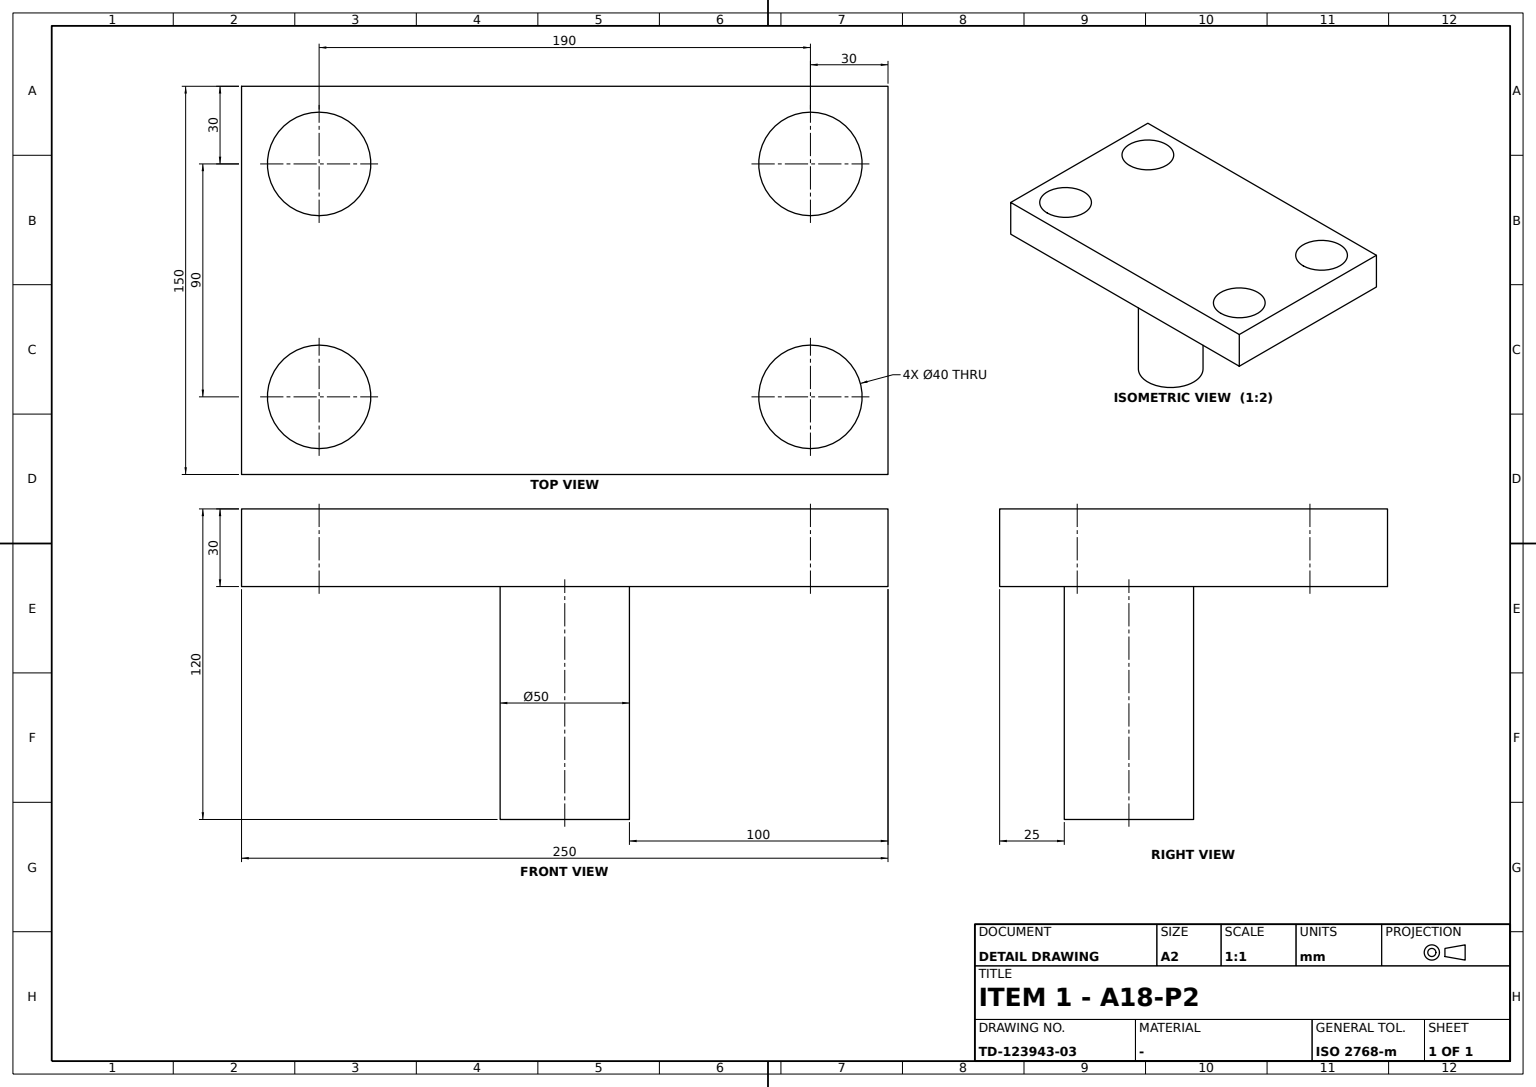
ISO-10303-21;
HEADER;
FILE_DESCRIPTION((''),'2;1');
FILE_NAME('','',(''),(''),'','','');
FILE_SCHEMA(('AUTOMOTIVE_DESIGN'));
ENDSEC;
DATA;
#1=APPLICATION_CONTEXT('');
#2=PRODUCT_CONTEXT('',#1,'mechanical');
#3=PRODUCT('','','',(#2));
#4=PRODUCT_DEFINITION_FORMATION('','',#3);
#5=PRODUCT_DEFINITION_CONTEXT('',#1,'design');
#6=PRODUCT_DEFINITION('','',#4,#5);
#7=PRODUCT_DEFINITION_SHAPE('','',#6);
#8=(LENGTH_UNIT()NAMED_UNIT(*)SI_UNIT(.MILLI.,.METRE.));
#9=(NAMED_UNIT(*)PLANE_ANGLE_UNIT()SI_UNIT($,.RADIAN.));
#10=(NAMED_UNIT(*)SI_UNIT($,.STERADIAN.)SOLID_ANGLE_UNIT());
#11=UNCERTAINTY_MEASURE_WITH_UNIT(LENGTH_MEASURE(0.005),#8,'distance_accuracy_value','');
#12=(GEOMETRIC_REPRESENTATION_CONTEXT(3)GLOBAL_UNCERTAINTY_ASSIGNED_CONTEXT((#11))GLOBAL_UNIT_ASSIGNED_CONTEXT((#8,#9,#10))REPRESENTATION_CONTEXT('',''));
#13=CARTESIAN_POINT('',(65.,95.,-15.));
#14=VERTEX_POINT('',#13);
#15=CARTESIAN_POINT('',(45.,95.,-15.));
#16=DIRECTION('',(0.,0.,1.));
#17=DIRECTION('',(1.,0.,0.));
#18=AXIS2_PLACEMENT_3D('',#15,#16,#17);
#19=CIRCLE('',#18,20.);
#20=EDGE_CURVE('',#14,#14,#19,.F.);
#21=ORIENTED_EDGE('',*,*,#20,.T.);
#22=EDGE_LOOP('',(#21));
#23=FACE_BOUND('',#22,.T.);
#24=CARTESIAN_POINT('',(65.,95.,15.));
#25=VERTEX_POINT('',#24);
#26=CARTESIAN_POINT('',(45.,95.,15.));
#27=AXIS2_PLACEMENT_3D('',#26,#16,#17);
#28=CIRCLE('',#27,20.);
#29=EDGE_CURVE('',#25,#25,#28,.T.);
#30=ORIENTED_EDGE('',*,*,#29,.T.);
#31=EDGE_LOOP('',(#30));
#32=FACE_BOUND('',#31,.T.);
#33=CARTESIAN_POINT('',(45.,95.,14.9));
#34=DIRECTION('',(0.,0.,-1.));
#35=AXIS2_PLACEMENT_3D('',#33,#34,#17);
#36=CYLINDRICAL_SURFACE('',#35,20.);
#37=ADVANCED_FACE('',(#23,#32),#36,.F.);
#38=CARTESIAN_POINT('',(-25.,-95.,15.));
#39=VERTEX_POINT('',#38);
#40=CARTESIAN_POINT('',(-45.,-95.,15.));
#41=AXIS2_PLACEMENT_3D('',#40,#16,#17);
#42=CIRCLE('',#41,20.);
#43=EDGE_CURVE('',#39,#39,#42,.T.);
#44=ORIENTED_EDGE('',*,*,#43,.T.);
#45=EDGE_LOOP('',(#44));
#46=FACE_BOUND('',#45,.T.);
#47=CARTESIAN_POINT('',(-25.,-95.,-15.));
#48=VERTEX_POINT('',#47);
#49=CARTESIAN_POINT('',(-45.,-95.,-15.));
#50=AXIS2_PLACEMENT_3D('',#49,#16,#17);
#51=CIRCLE('',#50,20.);
#52=EDGE_CURVE('',#48,#48,#51,.F.);
#53=ORIENTED_EDGE('',*,*,#52,.T.);
#54=EDGE_LOOP('',(#53));
#55=FACE_BOUND('',#54,.T.);
#56=CARTESIAN_POINT('',(-45.,-95.,14.9));
#57=AXIS2_PLACEMENT_3D('',#56,#34,#17);
#58=CYLINDRICAL_SURFACE('',#57,20.);
#59=ADVANCED_FACE('',(#46,#55),#58,.F.);
#60=CARTESIAN_POINT('',(-25.,95.,15.));
#61=VERTEX_POINT('',#60);
#62=CARTESIAN_POINT('',(-45.,95.,15.));
#63=AXIS2_PLACEMENT_3D('',#62,#16,#17);
#64=CIRCLE('',#63,20.);
#65=EDGE_CURVE('',#61,#61,#64,.T.);
#66=ORIENTED_EDGE('',*,*,#65,.F.);
#67=EDGE_LOOP('',(#66));
#68=FACE_BOUND('',#67,.T.);
#69=ORIENTED_EDGE('',*,*,#43,.F.);
#70=EDGE_LOOP('',(#69));
#71=FACE_BOUND('',#70,.T.);
#72=CARTESIAN_POINT('',(75.,-125.,15.));
#73=VERTEX_POINT('',#72);
#74=CARTESIAN_POINT('',(-75.,-125.,15.));
#75=VERTEX_POINT('',#74);
#76=CARTESIAN_POINT('',(0.,-125.,15.));
#77=DIRECTION('',(-1.,0.,0.));
#78=VECTOR('',#77,1000.);
#79=LINE('',#76,#78);
#80=EDGE_CURVE('',#73,#75,#79,.T.);
#81=ORIENTED_EDGE('',*,*,#80,.F.);
#82=CARTESIAN_POINT('',(75.,125.,15.));
#83=VERTEX_POINT('',#82);
#84=CARTESIAN_POINT('',(75.,0.,15.));
#85=DIRECTION('',(0.,-1.,0.));
#86=VECTOR('',#85,1000.);
#87=LINE('',#84,#86);
#88=EDGE_CURVE('',#83,#73,#87,.T.);
#89=ORIENTED_EDGE('',*,*,#88,.F.);
#90=CARTESIAN_POINT('',(-75.,125.,15.));
#91=VERTEX_POINT('',#90);
#92=CARTESIAN_POINT('',(0.,125.,15.));
#93=VECTOR('',#17,1000.);
#94=LINE('',#92,#93);
#95=EDGE_CURVE('',#91,#83,#94,.T.);
#96=ORIENTED_EDGE('',*,*,#95,.F.);
#97=CARTESIAN_POINT('',(-75.,0.,15.));
#98=DIRECTION('',(0.,1.,0.));
#99=VECTOR('',#98,1000.);
#100=LINE('',#97,#99);
#101=EDGE_CURVE('',#75,#91,#100,.T.);
#102=ORIENTED_EDGE('',*,*,#101,.F.);
#103=EDGE_LOOP('',(#81,#89,#96,#102));
#104=FACE_BOUND('',#103,.T.);
#105=CARTESIAN_POINT('',(65.,-95.,15.));
#106=VERTEX_POINT('',#105);
#107=CARTESIAN_POINT('',(45.,-95.,15.));
#108=AXIS2_PLACEMENT_3D('',#107,#16,#17);
#109=CIRCLE('',#108,20.);
#110=EDGE_CURVE('',#106,#106,#109,.T.);
#111=ORIENTED_EDGE('',*,*,#110,.F.);
#112=EDGE_LOOP('',(#111));
#113=FACE_BOUND('',#112,.T.);
#114=ORIENTED_EDGE('',*,*,#29,.F.);
#115=EDGE_LOOP('',(#114));
#116=FACE_BOUND('',#115,.T.);
#117=CARTESIAN_POINT('',(0.,0.,15.));
#118=AXIS2_PLACEMENT_3D('',#117,#16,#98);
#119=PLANE('',#118);
#120=ADVANCED_FACE('',(#68,#71,#104,#113,#116),#119,.T.);
#121=ORIENTED_EDGE('',*,*,#101,.T.);
#122=CARTESIAN_POINT('',(-75.,125.,-15.));
#123=VERTEX_POINT('',#122);
#124=CARTESIAN_POINT('',(-75.,125.,0.));
#125=VECTOR('',#16,1000.);
#126=LINE('',#124,#125);
#127=EDGE_CURVE('',#123,#91,#126,.T.);
#128=ORIENTED_EDGE('',*,*,#127,.F.);
#129=CARTESIAN_POINT('',(-75.,-125.,-15.));
#130=VERTEX_POINT('',#129);
#131=CARTESIAN_POINT('',(-75.,0.,-15.));
#132=LINE('',#131,#99);
#133=EDGE_CURVE('',#130,#123,#132,.T.);
#134=ORIENTED_EDGE('',*,*,#133,.F.);
#135=CARTESIAN_POINT('',(-75.,-125.,0.));
#136=LINE('',#135,#125);
#137=EDGE_CURVE('',#130,#75,#136,.T.);
#138=ORIENTED_EDGE('',*,*,#137,.T.);
#139=EDGE_LOOP('',(#121,#128,#134,#138));
#140=FACE_BOUND('',#139,.T.);
#141=AXIS2_PLACEMENT_3D('',#135,#17,#98);
#142=PLANE('',#141);
#143=ADVANCED_FACE('',(#140),#142,.F.);
#144=ORIENTED_EDGE('',*,*,#110,.T.);
#145=EDGE_LOOP('',(#144));
#146=FACE_BOUND('',#145,.T.);
#147=CARTESIAN_POINT('',(65.,-95.,-15.));
#148=VERTEX_POINT('',#147);
#149=CARTESIAN_POINT('',(45.,-95.,-15.));
#150=AXIS2_PLACEMENT_3D('',#149,#16,#17);
#151=CIRCLE('',#150,20.);
#152=EDGE_CURVE('',#148,#148,#151,.F.);
#153=ORIENTED_EDGE('',*,*,#152,.T.);
#154=EDGE_LOOP('',(#153));
#155=FACE_BOUND('',#154,.T.);
#156=CARTESIAN_POINT('',(45.,-95.,14.9));
#157=AXIS2_PLACEMENT_3D('',#156,#34,#17);
#158=CYLINDRICAL_SURFACE('',#157,20.);
#159=ADVANCED_FACE('',(#146,#155),#158,.F.);
#160=CARTESIAN_POINT('',(75.,-125.,-15.));
#161=VERTEX_POINT('',#160);
#162=CARTESIAN_POINT('',(75.,-125.,0.));
#163=LINE('',#162,#125);
#164=EDGE_CURVE('',#161,#73,#163,.T.);
#165=ORIENTED_EDGE('',*,*,#164,.T.);
#166=ORIENTED_EDGE('',*,*,#80,.T.);
#167=ORIENTED_EDGE('',*,*,#137,.F.);
#168=CARTESIAN_POINT('',(0.,-125.,-15.));
#169=LINE('',#168,#78);
#170=EDGE_CURVE('',#161,#130,#169,.T.);
#171=ORIENTED_EDGE('',*,*,#170,.F.);
#172=EDGE_LOOP('',(#165,#166,#167,#171));
#173=FACE_BOUND('',#172,.T.);
#174=AXIS2_PLACEMENT_3D('',#162,#98,#77);
#175=PLANE('',#174);
#176=ADVANCED_FACE('',(#173),#175,.F.);
#177=CARTESIAN_POINT('',(0.,0.,-105.));
#178=VERTEX_POINT('',#177);
#179=CARTESIAN_POINT('',(25.,0.,-105.));
#180=AXIS2_PLACEMENT_3D('',#179,#34,#77);
#181=CIRCLE('',#180,25.);
#182=EDGE_CURVE('',#178,#178,#181,.T.);
#183=ORIENTED_EDGE('',*,*,#182,.T.);
#184=EDGE_LOOP('',(#183));
#185=FACE_BOUND('',#184,.T.);
#186=AXIS2_PLACEMENT_3D('',#177,#34,#98);
#187=PLANE('',#186);
#188=ADVANCED_FACE('',(#185),#187,.T.);
#189=CARTESIAN_POINT('',(75.,125.,-15.));
#190=VERTEX_POINT('',#189);
#191=CARTESIAN_POINT('',(75.,0.,-15.));
#192=LINE('',#191,#86);
#193=EDGE_CURVE('',#190,#161,#192,.T.);
#194=ORIENTED_EDGE('',*,*,#193,.F.);
#195=CARTESIAN_POINT('',(75.,125.,0.));
#196=LINE('',#195,#125);
#197=EDGE_CURVE('',#190,#83,#196,.T.);
#198=ORIENTED_EDGE('',*,*,#197,.T.);
#199=ORIENTED_EDGE('',*,*,#88,.T.);
#200=ORIENTED_EDGE('',*,*,#164,.F.);
#201=EDGE_LOOP('',(#194,#198,#199,#200));
#202=FACE_BOUND('',#201,.T.);
#203=AXIS2_PLACEMENT_3D('',#195,#77,#85);
#204=PLANE('',#203);
#205=ADVANCED_FACE('',(#202),#204,.F.);
#206=CARTESIAN_POINT('',(50.,0.,-15.));
#207=VERTEX_POINT('',#206);
#208=CARTESIAN_POINT('',(25.,0.,-15.));
#209=AXIS2_PLACEMENT_3D('',#208,#16,#17);
#210=CIRCLE('',#209,25.);
#211=EDGE_CURVE('',#207,#207,#210,.F.);
#212=ORIENTED_EDGE('',*,*,#211,.T.);
#213=EDGE_LOOP('',(#212));
#214=FACE_BOUND('',#213,.T.);
#215=ORIENTED_EDGE('',*,*,#182,.F.);
#216=EDGE_LOOP('',(#215));
#217=FACE_BOUND('',#216,.T.);
#218=CARTESIAN_POINT('',(25.,0.,-60.));
#219=AXIS2_PLACEMENT_3D('',#218,#34,#98);
#220=CYLINDRICAL_SURFACE('',#219,25.);
#221=ADVANCED_FACE('',(#214,#217),#220,.T.);
#222=ORIENTED_EDGE('',*,*,#197,.F.);
#223=CARTESIAN_POINT('',(0.,125.,-15.));
#224=LINE('',#223,#93);
#225=EDGE_CURVE('',#123,#190,#224,.T.);
#226=ORIENTED_EDGE('',*,*,#225,.F.);
#227=ORIENTED_EDGE('',*,*,#127,.T.);
#228=ORIENTED_EDGE('',*,*,#95,.T.);
#229=EDGE_LOOP('',(#222,#226,#227,#228));
#230=FACE_BOUND('',#229,.T.);
#231=AXIS2_PLACEMENT_3D('',#124,#85,#17);
#232=PLANE('',#231);
#233=ADVANCED_FACE('',(#230),#232,.F.);
#234=ORIENTED_EDGE('',*,*,#65,.T.);
#235=EDGE_LOOP('',(#234));
#236=FACE_BOUND('',#235,.T.);
#237=CARTESIAN_POINT('',(-25.,95.,-15.));
#238=VERTEX_POINT('',#237);
#239=CARTESIAN_POINT('',(-45.,95.,-15.));
#240=AXIS2_PLACEMENT_3D('',#239,#16,#17);
#241=CIRCLE('',#240,20.);
#242=EDGE_CURVE('',#238,#238,#241,.F.);
#243=ORIENTED_EDGE('',*,*,#242,.T.);
#244=EDGE_LOOP('',(#243));
#245=FACE_BOUND('',#244,.T.);
#246=CARTESIAN_POINT('',(-45.,95.,14.9));
#247=AXIS2_PLACEMENT_3D('',#246,#34,#17);
#248=CYLINDRICAL_SURFACE('',#247,20.);
#249=ADVANCED_FACE('',(#236,#245),#248,.F.);
#250=ORIENTED_EDGE('',*,*,#152,.F.);
#251=EDGE_LOOP('',(#250));
#252=FACE_BOUND('',#251,.T.);
#253=ORIENTED_EDGE('',*,*,#52,.F.);
#254=EDGE_LOOP('',(#253));
#255=FACE_BOUND('',#254,.T.);
#256=ORIENTED_EDGE('',*,*,#211,.F.);
#257=EDGE_LOOP('',(#256));
#258=FACE_BOUND('',#257,.T.);
#259=ORIENTED_EDGE('',*,*,#242,.F.);
#260=EDGE_LOOP('',(#259));
#261=FACE_BOUND('',#260,.T.);
#262=ORIENTED_EDGE('',*,*,#20,.F.);
#263=EDGE_LOOP('',(#262));
#264=FACE_BOUND('',#263,.T.);
#265=ORIENTED_EDGE('',*,*,#133,.T.);
#266=ORIENTED_EDGE('',*,*,#225,.T.);
#267=ORIENTED_EDGE('',*,*,#193,.T.);
#268=ORIENTED_EDGE('',*,*,#170,.T.);
#269=EDGE_LOOP('',(#265,#266,#267,#268));
#270=FACE_BOUND('',#269,.T.);
#271=CARTESIAN_POINT('',(0.,0.,-15.));
#272=AXIS2_PLACEMENT_3D('',#271,#16,#98);
#273=PLANE('',#272);
#274=ADVANCED_FACE('',(#252,#255,#258,#261,#264,#270),#273,.F.);
#275=CLOSED_SHELL('',(#37,#59,#120,#143,#159,#176,#188,#205,#221,#233,#249,#274));
#276=MANIFOLD_SOLID_BREP('',#275);
#277=ADVANCED_BREP_SHAPE_REPRESENTATION('',(#276),#12);
#278=SHAPE_DEFINITION_REPRESENTATION(#7,#277);
ENDSEC;
END-ISO-10303-21;
